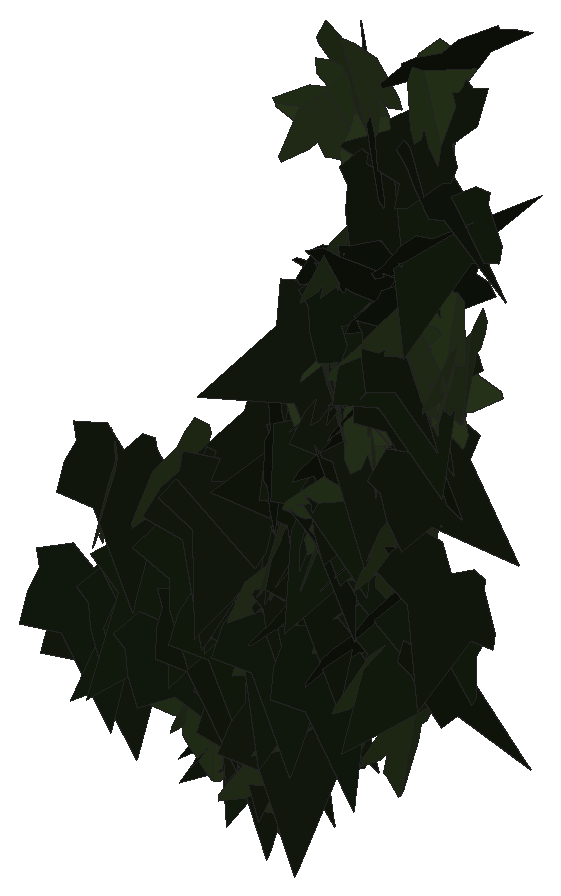
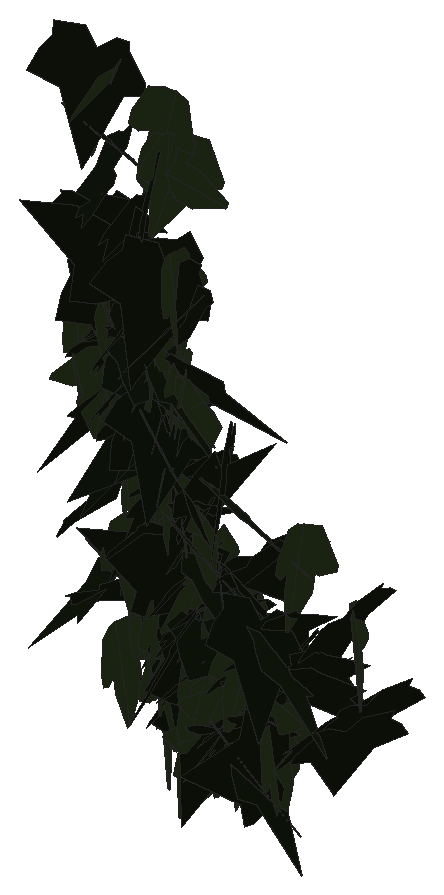
# SketchUp Ruby script. Lengths in inches.
U = 1.inch
M = Sketchup.active_model
def pt(a) = Geom::Point3d.new(a.map { |v| v * U })
def face(e, loops, mat)
  f = e.add_face(loops[0].map { |a| pt(a) })
  loops[1..].each { |l| e.add_face(l.map { |a| pt(a) }).erase! }
  f.material = f.back_material = mat if mat
  f
end
# faces: each face lists its corners as indices into pts; further lists are holes
def faces(e, pts, list, mat = nil) = list.each { |f| face(e, (f[0].is_a?(Array) ? f : [f]).map { |l| l.map { |i| pts[i] } }, mat) }
# xy, xz, yz: faces in a plane at the given z, y or x. An outline is a flat list of corners, or four numbers for a rectangle; further outlines are holes
def ring(l) = l.size == 4 ? [[l[0], l[1]], [l[2], l[1]], [l[2], l[3]], [l[0], l[3]]] : l.each_slice(2).to_a
def flat(e, list, mat, &to3) = list.each { |f| face(e, (f[0].is_a?(Array) ? f : [f]).map { |l| ring(l).map { |u, v| to3.(u, v) } }, mat) }
def xy(e, z, list, mat = nil) = flat(e, list, mat) { |x, y| [x, y, z] }
def xz(e, y, list, mat = nil) = flat(e, list, mat) { |x, z| [x, y, z] }
def yz(e, x, list, mat = nil) = flat(e, list, mat) { |y, z| [x, y, z] }
def lines(e, pts, list) = list.each { |a, b| e.add_line(pt(pts[a]), pt(pts[b])) }
# prism: a flat outline (further loops are holes) pulled along v
def prism(e, loops, v, mat = nil)
  f = face(e, loops, mat); d = Geom::Vector3d.new(v.map { |x| x * U })
  f.pushpull(f.normal.samedirection?(d) ? d.length : -d.length)
end
def box(e, o, s, mat = nil) = prism(e, [[o, [o[0] + s[0], o[1], o[2]], [o[0] + s[0], o[1] + s[1], o[2]], [o[0], o[1] + s[1], o[2]]]], [0, 0, s[2]], mat)
def at(x, y, z, deg = 0) = Geom::Transformation.translation(pt([x, y, z])) * Geom::Transformation.rotation(ORIGIN, Z_AXIS, deg.degrees)
def axes(o, x, y, z) = Geom::Transformation.new([*x, 0, *y, 0, *z, 0, *pt(o).to_a, 1])
def part(name) = M.definitions.add(name)
# library, detail: a bought-in or finely detailed component or shape, given as its bounding box
def library(name, o, s) = part(name).tap { |d| box(d.entities, o, s) }
def detail(e, o, s) = box(e.add_group.entities, o, s)
def put(e, d, t, mat = nil) = e.add_instance(d, t).tap { |i| i.material = mat if mat }
def group(e, t, mat = nil) = e.add_group.tap { |g| g.transformation = t; g.material = mat if mat }.entities
root = M.entities
M.materials.add("efeu1").color = [18, 25, 13]
M.materials.add("efeu2").color = [43, 57, 29]
c1 = part("ivyleaf_9")
p = [[1.54,2.16,1.25],[1.36,2.04,1.19],[-0.21,0.99,0.68],[-0.71,1.11,0.82],[-0.85,0.86,0.67],[-0.8,0.17,0.21],
  [-0.9,-0.01,0.1],[-0.67,-0.16,-0.02],[-0.08,-0.08,-0.05],[-0.03,-0.6,-0.4],[0.65,-0.88,-0.66],[0.83,-0.6,-0.49],
  [1.29,-0.42,-0.43],[1.8125,-0.07,-0.26],[1.21,0.44,0.15]]
faces(c1.entities,p,[[0,1,2,3,4,5,6,7,8,9,10,11,12,13,14]],"efeu1")
c2 = part("ivyleaf_10")
p = [[0,0.5,-0.03],[-0.0625,2.02,-0.43],[-0.19,2.01,-0.46],[-0.54,1.05,-0.29],[-0.52,0.625,-0.18],[-0.83,0.76,-0.28],
  [-1.16,0.64,-0.33],[-1.15,0.33,-0.24],[-0.77,-0.39,0.02],[-0.3,-0.51,0.16],[0.04,-0.48,0.23],[-0.02,2.01,-0.4375],
  [-0.06,2.01,-0.43],[0.04,-0.49,0.23],[0.67,-0.49,0.14],[1.38,0.36,-0.2],[1.375,0.51,-0.24],[0.81,0.65,-0.19],
  [0.62,0.59,-0.15],[0.6,1.09,-0.28],[0.5,1.23,-0.31]]
faces(c2.entities,p,[[0,1,2,3,4,5,6,7,8,9,10],[11,12,0,13,14,15,16,17,18,19,20]],"efeu2")
put(root,c1,axes([18.89,223.27,236.14],[-0.04259,-0.46339,0.18291],[-0.00233,-0.18339,-0.46515],[0.49818,-0.04048,0.01346]))
put(root,c1,axes([16.4,223.18,236.18],[-0.16822,-0.47035,-0.02179],[0.00609,0.02097,-0.49952],[0.47081,-0.16833,-0.00132]))
put(root,c2,axes([18.05,222.875,241.56],[-0.47923,0.13975,0.0285],[-0.0265,0.01093,-0.49918],[-0.14015,-0.47995,-0.00306]))
put(root,c2,axes([18.96,222.88,241.63],[-0.08504,0.49177,0.03045],[-0.02048,0.02735,-0.49883],[-0.49229,-0.08609,0.01549]))
put(root,c2,axes([17.86,222.85,241.02],[-0.1686,-0.41214,-0.22742],[0.10159,0.20401,-0.44504],[0.45962,-0.19627,0.01494]))
put(root,c1,axes([16.06,223.15,234.75],[0.16216,-0.47279,0.01329],[0.00406,-0.01265,-0.49982],[0.47296,0.16221,-0.00027]))
put(root,c1,axes([19.13,222.9375,240.99],[-0.34609,0.289,0.21611],[-0.22801,0.05696,-0.44132],[-0.2797,-0.40403,0.09236]))
put(root,c1,axes([16.45,223.32,236.08],[-0.16606,-0.45705,0.1163],[-0.00782,-0.12061,-0.48517],[0.47155,-0.16296,0.03291]))
put(root,c1,axes([17.52,223.16,234.87],[0.1089,-0.48718,-0.02825],[-0.00368,0.02812,-0.49919],[0.48798,0.10893,0.00254]))
put(root,c1,axes([18.89,223.2,240.14],[-0.37292,-0.28196,-0.17729],[0.1629,0.07774,-0.46628],[0.29051,-0.40553,0.03388]))
put(root,c1,axes([17.6,223.11,238.21],[-0.46382,0.08623,0.16563],[-0.16833,-0.0011,-0.47081],[-0.08083,-0.49251,0.03005]))
put(root,c1,axes([17.26,223.41,236.58],[-0.09097,-0.12894,0.47445],[-0.26115,-0.39613,-0.15773],[0.41656,-0.2765,0.00473]))
put(root,c1,axes([17.02,223.22,235.05],[-0.03294,-0.49674,-0.04649],[0.00796,0.04606,-0.49781],[0.49885,-0.03354,0.00487]))
put(root,c1,axes([17.81,222.82,239.27],[0.48605,0.02197,0.11522],[0.11077,0.07552,-0.48169],[-0.03857,0.49378,0.06854]))
put(root,c1,axes([17.16,223.23,234.06],[-0.09078,-0.48679,-0.06926],[0.01521,0.06761,-0.49517],[0.49145,-0.09201,0.00253]))
put(root,c1,axes([18.3125,223.04,240.35],[0.19522,-0.41536,-0.19841],[-0.0973,0.17341,-0.45876],[0.44991,0.21773,-0.01312]))
put(root,c2,axes([17.78,222.89,238.08],[-0.30918,0.36745,0.13923],[-0.11904,0.08125,-0.47878],[-0.37448,-0.32921,0.03724]))
put(root,c2,axes([17.81,223.03,239.46],[0.10901,-0.47988,-0.08851],[-0.01001,0.08848,-0.49201],[0.48787,0.10904,0.00968]))
put(root,c1,axes([18.78,223.05,240.58],[0.37507,-0.32818,-0.04024],[-0.02786,0.02928,-0.49836],[0.32946,0.37609,0.00368]))
put(root,c1,axes([17.15,222.8125,237.27],[0.15442,-0.07908,-0.46894],[-0.42394,0.20051,-0.17341],[0.21548,0.45116,-0.00512]))
put(root,c2,axes([18.5625,223.21,238.84],[0.02609,-0.4772,0.14697],[0.01008,-0.14663,-0.47791],[0.49922,0.0279,0.00197]))
put(root,c1,axes([17.6,222.76,235.7],[-0.04982,0.46829,0.16799],[-0.11483,0.15345,-0.46181],[-0.48408,-0.0846,0.09226]))
put(root,c2,axes([18.05,223.03,240.875],[0.11917,-0.00664,-0.48555],[-0.47703,0.09189,-0.11833],[0.0908,0.49144,0.01557]))
put(root,c1,axes([18.0625,223.25,237.64],[-0.15114,-0.46766,-0.09196],[0.02758,0.08773,-0.49147],[0.47581,-0.15363,-0.00072]))
put(root,c1,axes([15.78,223.03,234.61],[0.20026,-0.40299,-0.21794],[0.0358,0.25089,-0.43101],[0.45674,0.15702,0.12934]))
put(root,c2,axes([18.34,223.17,238.44],[-0.10902,-0.47949,0.0906],[0.00004,-0.09284,-0.49131],[0.48797,-0.10712,0.02028]))
put(root,c2,axes([17.125,223.05,233.73],[-0.16127,-0.47037,-0.0524],[0.01969,0.04864,-0.49724],[0.47287,-0.16245,0.00284]))
put(root,c2,axes([18.6,223.04,238.64],[-0.42135,0.25183,-0.09511],[0.0705,-0.06727,-0.49041],[-0.2598,-0.42668,0.02118]))
put(root,c2,axes([17.79,223.24,236.69],[-0.13365,-0.44512,0.18441],[-0.02022,-0.18603,-0.46366],[0.48138,-0.13139,0.03173]))
put(root,c1,axes([18.46,223.17,238.52],[-0.05102,-0.45013,-0.21161],[0.08167,0.20225,-0.44992],[0.49064,-0.08048,0.05289]))
put(root,c1,axes([17.81,223.11,238.79],[0.23729,-0.42458,-0.11587],[0.00612,0.13481,-0.48145],[0.44006,0.22707,0.06917]))
put(root,c1,axes([14.71,223.23,234.73],[-0.02443,-0.48315,-0.12637],[0.01064,0.12599,-0.48375],[0.49929,-0.02632,0.00413]))
put(root,c1,axes([17.34,223.37,236.2],[0.17358,-0.39844,0.24722],[0.09141,-0.2298,-0.43455],[0.45991,0.19605,-0.00694]))
put(root,c1,axes([17.625,223.21,237.15],[0.31512,-0.38326,0.06177],[0.04005,-0.04703,-0.49617],[0.38613,0.31765,0.00106]))
put(root,c1,axes([18.77,222.95,237.52],[0.22404,-0.29117,-0.33916],[-0.06944,0.3521,-0.34815],[0.44157,0.2031,0.11733]))
put(root,c1,axes([15.69,223.38,234.99],[-0.40771,-0.28382,0.05677],[-0.04029,-0.04146,-0.49665],[0.28662,-0.40955,0.01094]))
put(root,c1,axes([18.37,223.16,238.67],[0.22258,-0.42549,-0.13935],[-0.07103,0.12009,-0.48014],[0.44206,0.23353,-0.00698]))
put(root,c2,axes([17.83,222.94,238.15],[-0.23804,0.39084,0.20144],[-0.1799,0.12245,-0.45016],[-0.40121,-0.28679,0.08233]))
put(root,c1,axes([16.93,223.4,234.94],[-0.12543,-0.48165,0.0477],[-0.00324,-0.04844,-0.49764],[0.484,-0.12515,0.00903]))
put(root,c1,axes([17.64,223.43,236.49],[-0.34607,-0.36087,-0.00188],[0.09136,-0.0851,-0.48416],[0.34912,-0.33545,0.12484]))
put(root,c2,axes([18.37,223.09,236.61],[0.11078,-0.47194,-0.12248],[0.0003,0.12567,-0.48395],[0.48757,0.10715,0.02812]))
put(root,c1,axes([18.22,223.16,238.35],[-0.31746,0.35976,-0.1407],[0.00291,-0.17988,-0.46651],[-0.38628,-0.29702,0.11211]))
put(root,c2,axes([18.89,223.24,238.9],[0.4164,-0.24817,0.12257],[0.11073,-0.05357,-0.48463],[0.25367,0.43075,0.01035]))
put(root,c1,axes([17.46,223.27,237.04],[0.01207,-0.48431,-0.12369],[0.10082,0.12355,-0.47389],[0.48958,-0.0135,0.10064]))
put(root,c2,axes([15.86,223.02,236.4375],[-0.01197,-0.45256,-0.21223],[0.03822,0.21084,-0.45176],[0.49839,-0.02704,0.02955]))
put(root,c1,axes([19.15,222.87,241.98],[0.1385,0.48034,-0.00966],[-0.07837,0.01267,-0.49366],[-0.474,0.13826,0.07879]))
put(root,c2,axes([18.1,223.2,237.94],[-0.15487,0.44851,-0.15764],[0.00086,-0.16553,-0.4718],[-0.47541,-0.14641,0.0505]))
put(root,c1,axes([15.64,223.39,234.82],[-0.4685,-0.16814,0.04732],[-0.03294,-0.04796,-0.4966],[0.17154,-0.46843,0.03386]))
put(root,c2,axes([18.36,223.17,238.45],[-0.45184,0.18308,-0.11098],[0.07275,-0.11246,-0.48173],[-0.20135,-0.45148,0.07499]))
put(root,c1,axes([18.25,223.3,238.05],[0.17615,-0.46662,-0.03517],[0.00208,0.03835,-0.49852],[0.46794,0.17548,0.01545]))
put(root,c1,axes([17.97,223.14,238.3],[-0.36465,0.3393,-0.0437],[0.03758,-0.02375,-0.49802],[-0.34003,-0.36649,-0.00818]))
put(root,c1,axes([18.29,223.01,240.32],[0.01782,-0.22404,0.44664],[-0.04302,0.44458,0.22472],[-0.49783,-0.04644,-0.00343]))
put(root,c2,axes([16.96,223.2,236.01],[0.23552,-0.43888,-0.04373],[0.04089,0.07109,-0.49323],[0.43915,0.22876,0.06938]))
put(root,c2,axes([17.97,223.21,238.01],[0.45673,0.17421,-0.10512],[-0.1154,0.00901,-0.48642],[-0.16758,0.46858,0.04844]))
put(root,c1,axes([18,223.1,237.43],[-0.03958,0.46461,-0.18049],[0.00684,-0.18053,-0.46622],[-0.49838,-0.03938,0.00793]))
put(root,c1,axes([16.1,223.5,235.39],[-0.25844,-0.42562,0.04533],[0.0179,-0.06365,-0.49561],[0.42765,-0.25455,0.04814]))
put(root,c1,axes([17.14,223.36,235.98],[-0.38937,0.20712,-0.23556],[0.13272,-0.23145,-0.42287],[-0.28421,-0.39183,0.12526]))
put(root,c1,axes([18.67,223.09,239.17],[0.06665,0.45873,-0.18742],[-0.02246,-0.18612,-0.46352],[-0.49503,0.0702,-0.00421]))
put(root,c1,axes([18.11,223.24,237.875],[-0.03285,-0.00715,-0.49887],[0.47339,0.15744,-0.03343],[0.15756,-0.47451,-0.00357]))
put(root,c1,axes([16.33,223.41,234.88],[-0.01084,-0.49756,-0.04809],[0.00076,0.04808,-0.49768],[0.49988,-0.01087,-0.00029]))
put(root,c2,axes([18.15,223.09,237.77],[0.03496,0.491,0.08772],[0.0122,0.08707,-0.49221],[-0.49863,0.03655,-0.00589]))
put(root,c2,axes([17.43,223.24,236.15],[0.23054,-0.44092,-0.04943],[0.00784,0.05975,-0.49636],[0.44361,0.22809,0.03447]))
put(root,c2,axes([16.19,223.21,233.97],[-0.43528,-0.24111,0.04892],[-0.04037,-0.02807,-0.49758],[0.24269,-0.43712,0.00497]))
put(root,c1,axes([18.3,223.03,238.15],[-0.12519,0.48407,0.00088],[0.00437,0.00204,-0.49998],[-0.48405,-0.12518,-0.00474]))
put(root,c1,axes([17.28,223.44,235.7],[0.08435,-0.49166,0.03403],[-0.00013,-0.03455,-0.4988],[0.49283,0.08414,-0.00595]))
put(root,c1,axes([14.9,223.43,235.96],[0.03861,-0.49835,-0.0126],[-0.0097,0.01189,-0.49976],[0.49841,0.03884,-0.00875]))
put(root,c1,axes([18.63,222.98,239.44],[0.14719,0.45276,-0.15277],[0.05528,0.14265,0.47602],[0.47464,-0.15702,-0.00806]))
put(root,c1,axes([18.04,222.9375,235.4],[0.00389,0.48428,0.12433],[-0.00801,0.12437,-0.48422],[-0.49992,0.00177,0.00873]))
put(root,c1,axes([16.71,223.32,235.83],[-0.4793,0.14234,-0.00372],[0.00326,-0.00211,-0.49998],[-0.14235,-0.47931,0.00109]))
put(root,c2,axes([16.95,223.12,235.59],[-0.10149,-0.43534,-0.22401],[0.05862,0.21632,-0.44696],[0.48607,-0.11699,0.00713]))
put(root,c1,axes([18.4375,223.61,235.2],[-0.34735,-0.34109,0.11402],[0.01443,-0.1716,-0.46941],[0.35936,-0.32281,0.12906]))
put(root,c2,axes([18.03,223.32,234.9375],[0.08738,-0.49226,0.00679],[0.00111,-0.0067,-0.49995],[0.4923,0.08739,-0.00008]))
put(root,c2,axes([17.47,223.16,237.8],[0.30758,0.08886,0.38405],[0.33009,0.20824,-0.31254],[-0.21549,0.4458,0.06944]))
put(root,c1,axes([17.98,223.02,239.45],[0.24014,0.43731,-0.03312],[-0.01648,-0.02874,-0.4989],[-0.43825,0.2407,0.00061]))
put(root,c1,axes([16.49,223.52,233.82],[0.0347,-0.49731,0.0384],[0.00426,-0.0382,-0.49852],[0.49878,0.03493,0.00159]))
put(root,c2,axes([18.37,223.24,238.57],[-0.49902,-0.02926,0.01117],[-0.01089,-0.00515,-0.49985],[0.02937,-0.49912,0.0045]))
put(root,c1,axes([16.49,223.59,234.07],[-0.02805,-0.48699,0.10978],[0.0552,-0.1123,-0.48409],[0.49615,-0.01504,0.06006]))
put(root,c1,axes([14.86,223.4375,234.4],[-0.08086,-0.46579,-0.16279],[0.04125,0.158,-0.47258],[0.49169,-0.08985,0.01288]))
put(root,c2,axes([19.07,223.28,238.63],[0.07676,-0.47967,-0.11842],[-0.00092,0.1197,-0.48546],[0.49407,0.07475,0.01749]))
put(root,c2,axes([17.13,223.43,235.66],[0.02983,0.45226,-0.21112],[-0.0153,-0.21057,-0.45324],[-0.49887,0.03351,0.00128]))
put(root,c2,axes([18.63,223.23,238.05],[0.29223,0.39448,0.09483],[-0.00223,0.11843,-0.48577],[-0.40571,0.28349,0.07098]))
put(root,c2,axes([18.16,223.22,238.13],[-0.40751,0.28267,0.06354],[-0.05434,0.03313,-0.49593],[-0.28458,-0.4111,0.00372]))
put(root,c1,axes([16.83,223.38,236.96],[-0.43806,0.22636,0.08283],[-0.1039,-0.02227,-0.48858],[-0.2175,-0.44527,0.06655]))
put(root,c1,axes([16.59,223.52,234.66],[-0.38833,-0.27202,-0.15875],[0.12865,0.09303,-0.47412],[0.28748,-0.40908,-0.00226]))
put(root,c2,axes([17.7,223.3125,236.7],[-0.49452,0.04116,-0.06129],[0.05827,-0.03729,-0.49519],[-0.04534,-0.49691,0.03208]))
put(root,c2,axes([14.84,223.29,235.83],[0.25097,-0.39424,-0.17773],[-0.04622,0.17985,-0.46424],[0.42998,0.24945,0.05383]))
put(root,c1,axes([18.62,223.3,235.21],[0.39245,-0.2691,-0.15352],[-0.05986,0.17723,-0.46369],[0.30397,0.38233,0.10689]))
put(root,c1,axes([17.45,223.42,236.3125],[-0.42285,0.25179,0.08832],[-0.08655,0.02713,-0.4917],[-0.2524,-0.43112,0.02064]))
put(root,c2,axes([18.3,223.45,234.44],[0.03818,-0.49681,-0.04149],[0.0021,0.04177,-0.49825],[0.49854,0.03787,0.00527]))
put(root,c2,axes([17.22,223.43,236.33],[-0.44811,0.11368,-0.19045],[0.17454,-0.08415,-0.46093],[-0.13685,-0.47958,0.03573]))
put(root,c1,axes([17.875,223.22,237.49],[0.49936,0.02511,0.00233],[-0.00259,0.09694,-0.49051],[-0.02509,0.48987,0.09695]))
put(root,c1,axes([18.06,223.26,237.55],[0.44329,-0.08581,-0.21479],[-0.19339,0.11719,-0.44594],[0.12687,0.47844,0.0707]))
put(root,c1,axes([17.65,223.49,236.27],[0.05338,-0.44774,-0.21606],[0.01917,0.21899,-0.44908],[0.49677,0.03966,0.04054]))
put(root,c2,axes([16.23,223.44,233.73],[-0.30181,0.38512,-0.10292],[0.07746,-0.06997,-0.48898],[-0.39104,-0.3111,-0.01743]))
put(root,c1,axes([17.27,223.42,236.57],[-0.19965,0.32842,0.31981],[0.16397,-0.27458,0.38434],[0.42808,0.25835,0.00194]))
put(root,c1,axes([14.97,223.48,234.58],[0.21014,-0.41622,-0.18056],[0.041,0.2156,-0.44926],[0.45184,0.17401,0.12474]))
put(root,c2,axes([16.31,223.58,234.23],[-0.44051,-0.17488,0.15928],[-0.0982,-0.1711,-0.45943],[0.2152,-0.43605,0.1164]))
put(root,c1,axes([17.03,223.4,235.36],[0.23498,-0.35926,-0.25636],[-0.04667,0.26857,-0.41915],[0.43887,0.22092,0.09269]))
put(root,c1,axes([17,223.5,235.16],[-0.28141,0.38373,-0.15349],[0.00326,-0.18363,-0.46505],[-0.41328,-0.26274,0.10085]))
put(root,c1,axes([17.625,223.35,236.79],[0.18034,-0.30606,-0.35186],[-0.14374,0.3224,-0.35411],[0.44364,0.22887,0.0283]))
put(root,c2,axes([16.89,223.54,234.72],[-0.1026,-0.489,0.01873],[0.00313,-0.0198,-0.4996],[0.48935,-0.1024,0.00713]))
put(root,c1,axes([17.26,223.48,235.58],[0.20296,-0.07436,0.45086],[0.42353,-0.15459,-0.21616],[0.17154,0.46965,0.00023]))
put(root,c2,axes([17.6,223.45,236.92],[-0.25861,0.42269,0.06676],[-0.14551,-0.0135,-0.47817],[-0.40243,-0.26674,0.12999]))
put(root,c1,axes([16.48,223.76,234.03],[-0.32088,-0.37782,-0.06544],[0.05607,0.03818,-0.49538],[0.37933,-0.32526,0.01786]))
put(root,c2,axes([16.33,223.42,235.04],[-0.16907,-0.43181,-0.18696],[0.09824,0.16189,-0.46275],[0.46018,-0.19321,0.0301]))
put(root,c1,axes([17.74,223.25,237.71],[0.0982,0.48573,0.0665],[-0.01469,0.0707,-0.49476],[-0.49004,0.09521,0.02816]))
put(root,c1,axes([16.79,223.47,234.62],[0.372,0.32121,-0.09184],[0.07313,0.05582,0.49146],[0.32598,-0.37909,-0.00545]))
put(root,c2,axes([18.02,223.52,236.09],[-0.13751,-0.47461,-0.07638],[0.00787,0.0772,-0.49394],[0.48065,-0.13705,-0.01376]))
put(root,c2,axes([16.7,223.65,234.36],[-0.25907,-0.41156,0.11619],[-0.0209,-0.1235,-0.48406],[0.42714,-0.25566,0.04678]))
put(root,c2,axes([15.85,223.57,233.9375],[0.10656,-0.48607,-0.04884],[0.00929,0.052,-0.4972],[0.48843,0.10506,0.02011]))
put(root,c1,axes([16.89,223.57,234.71],[0.21241,-0.41471,-0.18138],[-0.00148,0.19973,-0.45837],[0.45264,0.19526,0.08362]))
put(root,c2,axes([17.38,223.54,234.52],[-0.17029,-0.46545,-0.06599],[0.00767,0.06743,-0.49537],[0.47005,-0.16972,-0.01582]))
put(root,c2,axes([17.53,223.51,235.125],[-0.03976,-0.46924,-0.16802],[0.05287,0.16364,-0.4695],[0.4956,-0.0551,0.0366]))
put(root,c1,axes([16.55,223.63,233.82],[-0.44902,0.2198,0.00809],[-0.00484,0.00851,-0.4999],[-0.2199,-0.44902,-0.00551]))
put(root,c2,axes([16.94,223.58,234.63],[-0.31921,0.38455,-0.01498],[0.00729,-0.01342,-0.49977],[-0.38477,-0.31928,0.00296]))
put(root,c1,axes([16.5,223.79,233.99],[0.23032,-0.4433,0.02093],[0.01978,-0.0133,-0.49943],[0.44335,0.23089,0.01141]))
put(root,c1,axes([17.27,223.49,235.69],[0.04006,0.01124,0.49827],[0.49603,0.04768,-0.04096],[-0.04843,0.49759,-0.00733]))
put(root,c2,axes([17.39,223.74,234.02],[0.33539,-0.36631,-0.0577],[0.0293,0.10373,-0.48824],[0.36967,0.32412,0.09105]))
put(root,c1,axes([15.8,223.6,235.2],[-0.28134,0.38751,0.14384],[-0.09561,0.10827,-0.47868],[-0.40213,-0.29684,0.01318]))
put(root,c1,axes([17.15,223.52,235.17],[0.28333,-0.13459,-0.38937],[-0.2697,0.29663,-0.29878],[0.31142,0.37934,0.09549]))
put(root,c1,axes([16.06,223.7,233.7],[-0.28053,0.41371,-0.01235],[0.00625,-0.01069,-0.49985],[-0.41384,-0.28059,0.00082]))
put(root,c2,axes([16.59,223.53,234.17],[0.08369,0.36409,0.33232],[0.07702,0.32327,-0.37358],[-0.48689,0.11372,-0.00198]))
put(root,c1,axes([16.08,223.56,235.52],[-0.00935,0.49903,0.02965],[0.00025,0.02966,-0.49912],[-0.49991,-0.00932,-0.00081]))
put(root,c1,axes([16.58,223.65,234.2],[0.40072,0.24571,-0.17045],[-0.18746,-0.01565,-0.46327],[-0.23299,0.43518,0.07958]))
put(root,c2,axes([16.58,223.67,233.78],[0.25091,0.32215,0.28856],[0.0137,0.32752,-0.37755],[-0.43227,0.19737,0.15553]))
put(root,c1,axes([15.84,223.68,233.69],[0.09143,0.12179,0.47624],[0.2845,0.38193,-0.15229],[-0.40087,0.29883,0.00054]))
